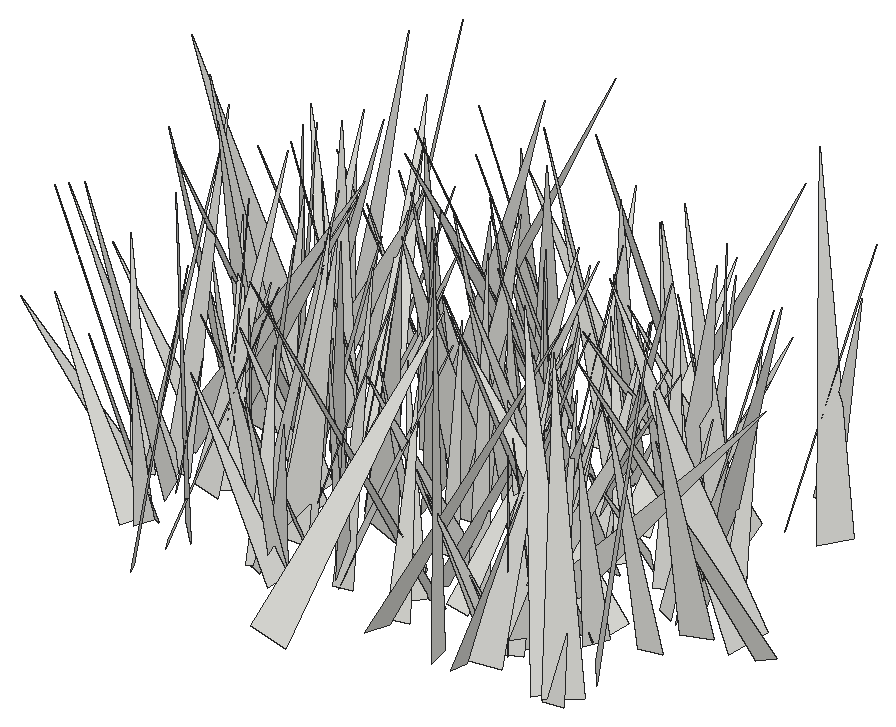
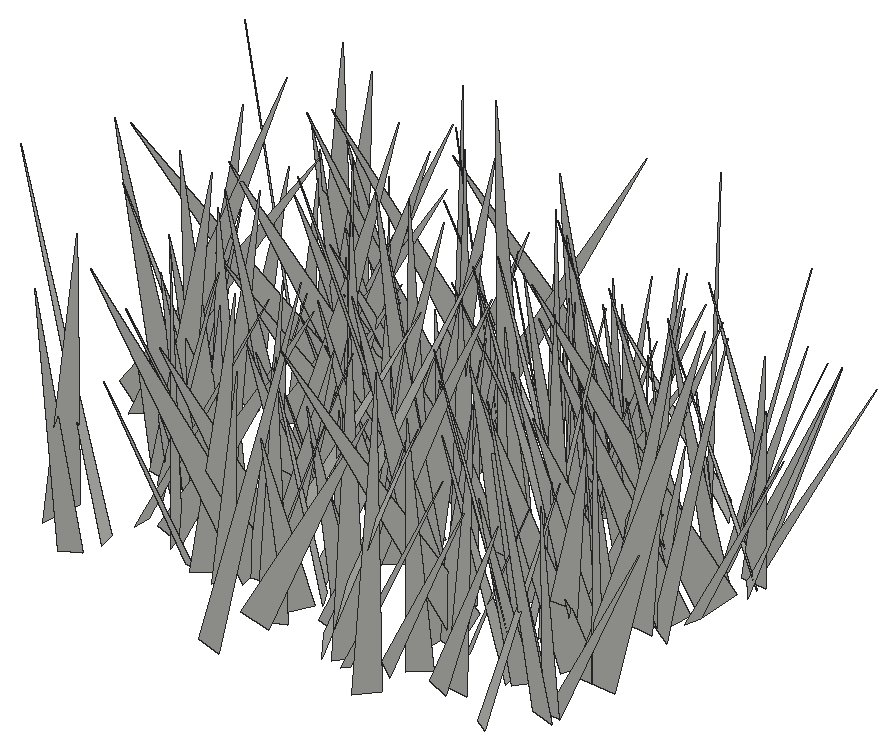
# SketchUp Ruby script. Lengths in inches.
U = 1.inch
M = Sketchup.active_model
def pt(a) = Geom::Point3d.new(a.map { |v| v * U })
def face(e, loops, mat)
  f = e.add_face(loops[0].map { |a| pt(a) })
  loops[1..].each { |l| e.add_face(l.map { |a| pt(a) }).erase! }
  f.material = f.back_material = mat if mat
  f
end
# faces: each face lists its corners as indices into pts; further lists are holes
def faces(e, pts, list, mat = nil) = list.each { |f| face(e, (f[0].is_a?(Array) ? f : [f]).map { |l| l.map { |i| pts[i] } }, mat) }
# xy, xz, yz: faces in a plane at the given z, y or x. An outline is a flat list of corners, or four numbers for a rectangle; further outlines are holes
def ring(l) = l.size == 4 ? [[l[0], l[1]], [l[2], l[1]], [l[2], l[3]], [l[0], l[3]]] : l.each_slice(2).to_a
def flat(e, list, mat, &to3) = list.each { |f| face(e, (f[0].is_a?(Array) ? f : [f]).map { |l| ring(l).map { |u, v| to3.(u, v) } }, mat) }
def xy(e, z, list, mat = nil) = flat(e, list, mat) { |x, y| [x, y, z] }
def xz(e, y, list, mat = nil) = flat(e, list, mat) { |x, z| [x, y, z] }
def yz(e, x, list, mat = nil) = flat(e, list, mat) { |y, z| [x, y, z] }
def lines(e, pts, list) = list.each { |a, b| e.add_line(pt(pts[a]), pt(pts[b])) }
# prism: a flat outline (further loops are holes) pulled along v
def prism(e, loops, v, mat = nil)
  f = face(e, loops, mat); d = Geom::Vector3d.new(v.map { |x| x * U })
  f.pushpull(f.normal.samedirection?(d) ? d.length : -d.length)
end
def box(e, o, s, mat = nil) = prism(e, [[o, [o[0] + s[0], o[1], o[2]], [o[0] + s[0], o[1] + s[1], o[2]], [o[0], o[1] + s[1], o[2]]]], [0, 0, s[2]], mat)
def at(x, y, z, deg = 0) = Geom::Transformation.translation(pt([x, y, z])) * Geom::Transformation.rotation(ORIGIN, Z_AXIS, deg.degrees)
def axes(o, x, y, z) = Geom::Transformation.new([*x, 0, *y, 0, *z, 0, *pt(o).to_a, 1])
def part(name) = M.definitions.add(name)
# library, detail: a bought-in or finely detailed component or shape, given as its bounding box
def library(name, o, s) = part(name).tap { |d| box(d.entities, o, s) }
def detail(e, o, s) = box(e.add_group.entities, o, s)
def put(e, d, t, mat = nil) = e.add_instance(d, t).tap { |i| i.material = mat if mat }
def group(e, t, mat = nil) = e.add_group.tap { |g| g.transformation = t; g.material = mat if mat }.entities
root = M.entities
c1 = part("fur_instance\#9")
p = [[0.8125,0,1.79],[0.67,-0.02,1.48],[0,-0.11,0],[0,0.11,0]]
faces(c1.entities,p,[[0,1,2,3]])
put(root,c1,axes([76.67,339.64,-27.1],[-0.73588,7.38124,0.25307],[6.98236,0.77818,-2.39362],[2.40696,-0.00075,7.02103]))
put(root,c1,axes([69.36,340.53,-27.1],[4.53649,3.63122,1.57008],[3.09166,-4.74451,2.04009],[-2.46831,0.73111,5.44092]))
put(root,c1,axes([74.26,343.21,-27.1],[-4.45422,0.97791,0.2811],[1.01486,4.3608,0.91044],[0.07343,-0.95002,4.4685]))
put(root,c1,axes([73.88,343.84,-27.1],[-3.9744,-0.24759,1.6573],[0.13335,4.20562,0.94807],[1.67038,-0.92483,3.8676]))
put(root,c1,axes([67.49,343.58,-27.1],[2.92591,-1.89098,1.19539],[-1.88086,-3.14489,-0.37117],[-1.21125,0.31559,3.46396]))
put(root,c1,axes([73.47,344.22,-27.1],[0.57309,-4.07864,0.58369],[-4.03575,-0.43699,0.90892],[0.82985,0.69149,4.01716]))
put(root,c1,axes([67.57,344.0625,-27.1],[-2.05359,-3.75931,0.63579],[-3.81243,2.01617,-0.39286],[-0.04503,0.74602,4.26559]))
put(root,c1,axes([88.39,342.84,-27.1],[-4.52139,5.22079,2.42729],[5.56937,4.74843,0.161],[1.45961,-1.94607,6.90462]))
put(root,c1,axes([67.04,343.47,-27.1],[-3.88022,2.75048,0.41463],[2.75578,3.70465,1.21426],[-0.37781,-1.22622,4.59857]))
put(root,c1,axes([69.24,344.07,-27.1],[-4.9247,-5.05159,2.9073],[-5.39927,5.38751,0.21521],[2.19519,1.91829,7.05159]))
put(root,c1,axes([80.1,345.62,-27.1],[-3.80092,-6.72254,0.0507],[-6.48684,3.65215,-2.05545],[-1.76524,1.05421,7.4441]))
put(root,c1,axes([82.68,342.42,-27.1],[-7.45834,-2.27512,2.73301],[-2.96816,7.48025,-1.87304],[1.95846,2.67246,7.56933]))
put(root,c1,axes([84.33,344.62,-27.1],[-3.42009,-2.62307,1.97794],[-2.56254,3.91671,0.76324],[2.05575,0.51835,4.24205]))
put(root,c1,axes([87.82,342.95,-27.1],[-6.04844,4.67756,1.28768],[4.75602,6.12308,0.0974],[0.95811,-0.86582,7.6455]))
put(root,c1,axes([75.96,345.09,-27.1],[3.91592,-0.46866,0.80636],[-0.26131,-3.89224,-0.99321],[-0.89531,-0.91384,3.81675]))
put(root,c1,axes([84.44,343.05,-27.1],[-2.07384,5.25709,1.74566],[5.26815,2.4479,-1.11335],[1.712,-1.16445,5.54061]))
put(root,c1,axes([88.37,342.28,-27.1],[1.19098,5.93826,0.851],[5.76454,-1.37303,1.51343],[-1.66049,-0.50738,5.86438]))
put(root,c1,axes([82.39,345.78,-27.1],[-3.37943,-0.96857,0.84627],[-0.6019,3.29348,1.36586],[1.13667,-1.13567,3.23931]))
put(root,c1,axes([73,343.66,-27.1],[-1.62337,4.08317,1.17277],[4.21606,1.70273,-0.09236],[0.52201,-1.05424,4.39307]))
put(root,c1,axes([82.14,345.75,-27.1],[0.37183,-3.94608,0.38846],[-3.8933,-0.43727,-0.71534],[-0.75144,0.31297,3.89847]))
put(root,c1,axes([65.42,346.04,-27.1],[-4.70731,-0.314,0.0439],[-0.28456,4.4722,1.47573],[0.13983,-1.46975,4.48103]))
put(root,c1,axes([79.5,342.71,-27.1],[7.73901,0.54751,0.09462],[0.50511,-7.48314,1.98706],[-0.23147,1.9758,7.49957]))
put(root,c1,axes([83.77,342.3125,-27.1],[6.82922,2.21825,1.16198],[1.82522,-6.72015,2.10172],[-1.71447,1.68168,6.86597]))
put(root,c1,axes([79.75,343.66,-27.1],[-0.43977,4.5707,0.64422],[4.59918,0.3789,0.45132],[-0.39225,-0.6818,4.56957]))
put(root,c1,axes([69.25,342.79,-27.1],[4.51704,3.2359,0.24642],[3.07452,-4.40221,1.45028],[-1.0388,1.04161,5.3639]))
put(root,c1,axes([66.73,346.16,-27.1],[-6.28754,-2.52373,1.27093],[-2.51372,6.41179,0.29625],[1.29062,0.19325,6.76865]))
put(root,c1,axes([75.96,344.84,-27.1],[4.98455,3.49636,0.32674],[3.50629,-4.92427,-0.79656],[0.19289,-0.83908,6.03621]))
put(root,c1,axes([88.13,345.15,-27.1],[5.88152,4.86813,2.28116],[5.13014,-6.09312,-0.22398],[-1.60749,-1.63397,7.63157]))
put(root,c1,axes([71.04,346.38,-27.1],[-4.89796,-0.50596,1.28828],[-0.38248,5.0478,0.52832],[1.33018,-0.4116,4.8956]))
put(root,c1,axes([66.65,346.67,-27.1],[3.46775,1.51161,0.84573],[1.722,-3.21287,-1.3182],[-0.18693,-1.55498,3.54578]))
put(root,c1,axes([72.72,346.24,-27.1],[2.84119,-6.18581,2.36185],[-6.62137,-2.65127,1.02137],[0.00779,2.57322,6.73004]))
put(root,c1,axes([75.22,345.87,-27.1],[1.82668,3.73793,1.95155],[3.99067,-2.21946,0.51574],[-1.36206,-1.48974,4.1283]))
put(root,c1,axes([84.125,346.46,-27.1],[-3.08736,-2.6391,1.38175],[-2.74426,3.29386,0.15946],[1.15895,0.7691,4.05847]))
put(root,c1,axes([72.91,343.4375,-27.1],[4.10406,6.33899,0.98584],[6.11766,-4.2195,1.66374],[-1.93105,0.10466,7.36601]))
put(root,c1,axes([73.32,346.04,-27.1],[-3.16767,-3.69393,0.44061],[-3.42422,2.66901,-2.24153],[-1.45395,1.76199,4.31912]))
put(root,c1,axes([86.07,347.09,-27.1],[-4.08084,-6.31933,0.93728],[-6.28934,3.77891,-1.90517],[-1.12095,1.80323,7.27719]))
put(root,c1,axes([78.36,346.8,-27.1],[-4.55771,-1.35516,1.4154],[-1.26006,4.77117,0.51063],[1.50069,-0.10962,4.72742]))
put(root,c1,axes([79.8125,348.23,-27.1],[1.26749,-5.25605,0.55346],[-5.00773,-1.37633,-1.60227],[-1.68968,0.13629,5.16385]))
put(root,c1,axes([84.64,344.8125,-27.1],[4.97283,-0.90694,1.68915],[-1.45035,-4.85051,1.66547],[-1.25389,2.01364,4.77261]))
put(root,c1,axes([86.66,347,-27.1],[3.6689,-2.8215,1.45683],[-2.81207,-3.92099,-0.512],[-1.47496,0.45716,4.59995]))
put(root,c1,axes([78.65,344.84,-27.1],[5.2038,5.70361,2.35891],[5.67233,-5.63566,1.11317],[-2.43315,-0.93989,7.64013]))
put(root,c1,axes([82.17,348.57,-27.1],[1.01842,-6.5564,0.3467],[-5.92672,-0.76709,2.90332],[2.82498,0.75429,5.9661]))
put(root,c1,axes([74.91,348.68,-27.1],[-0.13317,-8.12567,1.45261],[-7.87911,0.55826,2.40046],[2.46092,1.34765,7.76415]))
put(root,c1,axes([76.51,344.35,-27.1],[1.43264,6.02249,0.66756],[5.77311,-1.565,1.72927],[-1.84042,-0.22107,5.94411]))
put(root,c1,axes([79.24,345.34,-27.1],[-4.35702,1.54483,0.37411],[1.45493,4.3157,-0.87633],[0.64002,0.7059,4.53896]))
put(root,c1,axes([84.7,344.26,-27.1],[-5.37291,2.30629,0.61766],[1.96946,5.14098,-2.06404],[1.34972,1.6793,5.47055]))
put(root,c1,axes([65.08,346.9,-27.1],[-4.61833,-3.74237,0.73758],[-3.79853,4.40694,-1.4242],[-0.34716,1.56584,5.77113]))
put(root,c1,axes([84.61,346.72,-27.1],[2.40837,2.51325,1.53163],[2.71206,-2.66382,0.10655],[-1.14326,-1.0248,3.47927]))
put(root,c1,axes([72.71,346.01,-27.1],[-0.45657,6.34549,1.8425],[6.59681,0.54314,-0.23589],[0.37708,-1.81886,6.35752]))
put(root,c1,axes([66.14,347.15,-27.1],[-6.00367,-1.40851,0.07652],[-1.40991,5.98159,-0.51624],[-0.04369,0.52005,6.14503]))
put(root,c1,axes([71.98,348.5,-27.1],[-4.35378,0.44066,1.23045],[0.84047,4.2213,1.46212],[1.0009,-1.62788,4.12453]))
put(root,c1,axes([69.75,347.32,-27.1],[3.22406,2.21993,1.84513],[2.48282,-3.54361,-0.0749],[-1.47248,-1.11442,3.91371]))
put(root,c1,axes([88.67,347.77,-27.1],[-0.10037,-5.00985,1.67679],[-5.24561,-0.10471,-0.62683],[-0.62754,1.67652,4.9715]))
put(root,c1,axes([86.66,347.95,-27.1],[-6.39943,2.86094,0.01202],[2.71801,6.07041,2.2137],[-0.89308,-2.0256,6.65111]))
put(root,c1,axes([83.79,345.47,-27.1],[5.89458,-2.32049,1.52507],[-2.76984,-5.16651,2.8446],[-0.1962,3.22166,5.6603]))
put(root,c1,axes([65.08,346.52,-27.1],[-0.91318,4.58049,0.90258],[4.61205,0.74242,0.89849],[-0.72428,-1.04754,4.5834]))
put(root,c1,axes([80.95,345.74,-27.1],[-0.63847,4.33122,0.11328],[4.14955,0.64421,-1.24344],[1.2464,0.07394,4.19773]))
put(root,c1,axes([83.72,346.46,-27.1],[6.0984,-4.54505,0.22334],[-3.82324,-4.91501,4.37303],[2.46783,3.61705,6.22291]))
put(root,c1,axes([82.7,348.18,-27.1],[-2.40754,3.72637,1.88833],[4.14407,2.40561,0.53634],[0.52762,-1.89079,4.40391]))
put(root,c1,axes([79.36,346.64,-27.1],[5.44463,0.12063,0.24069],[0.04962,-5.23956,1.50366],[-0.26462,1.49964,5.23426]))
put(root,c1,axes([89.36,349.72,-27.1],[1.80262,-6.00522,1.15434],[-6.08405,-1.88243,-0.2921],[-0.61598,1.01901,6.26312]))
put(root,c1,axes([69.51,347.91,-27.1],[5.12051,1.66894,1.66295],[1.70709,-5.37015,0.13306],[-1.62376,-0.38277,5.38398]))
put(root,c1,axes([83.625,349.86,-27.1],[-0.04463,-6.97717,1.39975],[-6.92736,-0.27772,-1.60522],[-1.62845,1.37265,6.79015]))
put(root,c1,axes([80.7,347.34,-27.1],[1.55743,6.34801,1.89562],[6.44853,-1.89902,1.06134],[-1.51893,-1.55328,6.44953]))
put(root,c1,axes([69.49,348.87,-27.1],[3.75751,0.05108,0.3502],[0.07903,-3.76142,-0.29936],[-0.34497,-0.30538,3.74592]))
put(root,c1,axes([65.375,346.12,-27.1],[4.3588,4.87451,1.02077],[4.50794,-4.43827,1.9448],[-2.11691,0.58556,6.24322]))
put(root,c1,axes([92.48,350.04,-27.1],[-2.35699,-6.63901,0.53799],[-6.01099,1.87426,-3.2057],[-2.86948,1.52709,6.27339]))
put(root,c1,axes([67.8,346.96,-27.1],[1.8777,6.7714,0.98346],[6.8334,-1.90815,0.09124],[-0.35155,-0.923,7.02632]))
put(root,c1,axes([84.88,349.71,-27.1],[-2.69174,-3.80387,0.07847],[-3.66679,2.56798,-1.29661],[-1.01502,0.8106,4.47591]))
put(root,c1,axes([73.19,347.76,-27.1],[3.15484,4.86518,0.39731],[4.85003,-3.07066,-0.91053],[0.55227,-0.82578,5.72659]))
put(root,c1,axes([71.21,349.74,-27.1],[5.75664,2.23558,0.62086],[2.31995,-5.52205,-1.62697],[0.03364,-1.74108,5.95732]))
put(root,c1,axes([67.2,348.85,-27.1],[-4.37143,-2.8181,2.86453],[-3.24687,4.97094,-0.06453],[2.3675,1.61389,5.20067]))
put(root,c1,axes([83.4,347.96,-27.1],[1.4103,3.34023,0.25009],[3.32818,-1.428,0.30438],[-0.37801,-0.11091,3.61295]))
put(root,c1,axes([70.47,351.62,-27.1],[-2.5118,-6.70095,1.69222],[-6.07027,2.9998,2.86854],[3.30427,0.41708,6.55616]))
put(root,c1,axes([69.82,350.84,-27.1],[0.42063,-4.67833,0.35233],[-4.37367,-0.26302,1.72907],[1.69763,0.48155,4.36738]))
put(root,c1,axes([91.18,350.57,-27.1],[-7.69272,2.37823,1.5322],[2.71051,7.46743,2.01798],[0.8104,-2.40066,7.79498]))
put(root,c1,axes([83.34,351.62,-27.1],[-0.92127,-7.60318,0.93237],[-7.64439,0.85236,-0.60268],[-0.49091,0.99576,7.63504]))
put(root,c1,axes([71.22,349.92,-27.1],[-4.01235,0.08097,0.58825],[0.14386,4.03101,0.42638],[0.5761,-0.44265,3.99045]))
put(root,c1,axes([66.02,347.45,-27.1],[1.84085,7.01016,1.12106],[6.97031,-2.00445,1.08846],[-1.34679,-0.79226,7.16563]))
put(root,c1,axes([78.15,348.76,-27.1],[0.81104,4.54834,1.26147],[4.65262,-0.98593,0.56355],[-0.7949,-1.13006,4.58559]))
put(root,c1,axes([82.19,349.85,-27.1],[3.78368,4.97369,3.03573],[5.56614,-4.15585,-0.12867],[-1.72376,-2.50217,6.24798]))
put(root,c1,axes([68.58,347.65,-27.1],[-4.8792,2.06982,0.10093],[1.96371,4.70056,-1.46614],[0.66196,1.31208,5.09325]))
put(root,c1,axes([73.58,350,-27.1],[4.19942,-1.36084,1.21546],[-1.38514,-4.36301,-0.09922],[-1.1877,0.2767,4.41329]))
put(root,c1,axes([65.04,350.28,-27.1],[-4.32306,0.06447,0.02072],[0.06687,4.27292,0.65655],[0.01068,-0.65679,4.2734]))
put(root,c1,axes([74.94,351.86,-27.1],[7.73874,0.04549,1.82687],[0.5794,-7.60007,-2.26513],[-1.73315,-2.33761,7.39995]))
put(root,c1,axes([82.67,347.84,-27.1],[5.53562,0.75174,0.06867],[0.66774,-5.11345,2.14935],[-0.35205,2.12143,5.1564]))
put(root,c1,axes([75.98,353.14,-27.1],[6.63906,-4.24471,1.17982],[-3.75911,-6.57064,-2.48644],[-2.29753,-1.51516,7.47745]))
put(root,c1,axes([65.96,350.52,-27.1],[1.53162,3.70831,1.75315],[4.01532,-0.97314,-1.44953],[0.83802,-2.1148,3.74116]))
put(root,c1,axes([67.28,349.63,-27.1],[0.68239,3.8164,1.4602],[3.78451,-1.14857,1.23331],[-1.54098,-1.13076,3.67553]))
put(root,c1,axes([64.98,348.79,-27.1],[6.90826,-2.9112,0.5406],[-2.88435,-6.30625,2.89882],[0.66922,2.87186,6.91346]))
put(root,c1,axes([82.61,348.68,-27.1],[-6.55431,0.09701,1.7896],[-0.34688,6.588,-1.62754],[1.75834,1.66126,6.34976]))
put(root,c1,axes([88,352.11,-27.1],[-4.12038,-2.11418,1.50488],[-1.47976,4.23386,1.89649],[2.13184,-1.14743,4.225]))
put(root,c1,axes([71.97,349.47,-27.1],[3.98122,4.30027,2.75674],[4.211,-4.74141,1.31475],[-2.89126,-0.98426,5.71085]))
put(root,c1,axes([77.15,351.37,-27.1],[2.1882,-4.93746,0.79161],[-4.93819,-1.99768,1.19031],[0.78701,1.19336,5.26781]))
put(root,c1,axes([80.67,350.02,-27.1],[-3.32037,-5.8988,2.51801],[-6.36421,2.67847,-2.11746],[-0.7956,3.19234,6.42939]))
put(root,c1,axes([66.33,352.02,-27.1],[-0.95753,-7.17721,1.84222],[-7.39469,1.0444,0.22542],[0.47406,1.79439,7.23729]))
put(root,c1,axes([84.38,353.23,-27.1],[-2.58943,-3.13022,0.07236],[-2.65217,2.2427,2.10831],[1.66419,-1.2964,3.47253]))
put(root,c1,axes([73.65,348.23,-27.1],[5.66789,4.81372,1.80284],[4.22946,-5.89252,2.43659],[-2.92126,0.80836,7.02566]))
put(root,c1,axes([68.09,352.68,-27.1],[-3.16334,-6.14078,0.476],[-6.132,3.08971,-0.89149],[-0.57823,0.82883,6.8499]))
put(root,c1,axes([87.19,351.77,-27.1],[2.31724,-3.70248,0.25487],[-3.62607,-2.19471,1.08527],[0.79054,0.78602,4.23086]))
put(root,c1,axes([65.41,351.78,-27.1],[-3.32824,-5.52708,1.61735],[-5.74671,3.30884,-0.51825],[0.37393,1.65668,6.43096]))
put(root,c1,axes([87.33,350.34,-27.1],[1.79566,3.71313,0.76849],[3.77743,-1.82574,-0.00496],[-0.33004,-0.69403,4.12452]))
put(root,c1,axes([77.35,351.26,-27.1],[5.13352,5.29295,1.04527],[5.31008,-4.70157,-2.27141],[0.95446,-2.31104,7.01492]))
put(root,c1,axes([68.92,352.63,-27.1],[5.69332,3.04756,1.30745],[3.31373,-5.12843,-2.47574],[0.12746,-2.79687,5.96424]))
put(root,c1,axes([65.43,350.87,-27.1],[6.30652,-2.10429,0.15189],[-2.07978,-6.12031,1.56194],[0.35446,1.52876,6.46224]))
put(root,c1,axes([76.74,352.23,-27.1],[1.64053,-3.56149,0.70323],[-3.59089,-1.47867,0.88831],[0.53314,0.99969,3.81922]))
put(root,c1,axes([66.89,352.72,-27.1],[6.73753,-0.02978,4.19134],[0.53715,-7.86314,-0.91932],[-4.15689,-1.06433,6.67458]))
put(root,c1,axes([78.25,352.61,-27.1],[4.81176,-1.3762,1.70282],[-1.26945,-5.10354,-0.53746],[-1.78382,-0.0803,4.97575]))
put(root,c1,axes([86.23,351.98,-27.1],[-2.39493,4.93051,2.15105],[5.27679,2.61079,-0.10925],[1.04521,-1.88321,5.4803]))
put(root,c1,axes([87.83,350.42,-27.1],[5.27233,3.79468,0.9806],[3.62511,-5.34626,1.19781],[-1.48988,0.42019,6.38454]))
put(root,c1,axes([75.34,353.4,-27.1],[0.9927,-7.18833,2.00129],[-7.23058,-0.4281,2.04891],[1.84279,2.19257,6.96128]))
put(root,c1,axes([76.23,351.89,-27.1],[4.34648,-1.55951,0.20323],[-1.53377,-4.07129,1.56122],[0.34774,1.53551,4.34586]))
put(root,c1,axes([84.6,354.58,-27.1],[0.33482,-6.22736,0.74708],[-6.26175,-0.28913,0.39628],[0.3585,0.76592,6.22375]))
put(root,c1,axes([81.875,353.31,-27.1],[6.64605,0.23955,0.93352],[0.28653,-6.70181,-0.32012],[-0.92019,-0.35664,6.64266]))
put(root,c1,axes([72.625,354.61,-27.1],[0.91835,-4.65892,0.5996],[-4.68613,-0.86646,0.44487],[0.32448,0.67241,4.72768]))
put(root,c1,axes([69.25,354.91,-27.1],[-4.71687,-4.84842,1.35584],[-4.8132,4.8877,0.73342],[1.47602,0.44449,6.72444]))
put(root,c1,axes([86.52,354.12,-27.1],[7.28234,-1.08518,0.65082],[-1.04869,-7.30325,-0.44316],[-0.70811,-0.34428,7.3494]))
put(root,c1,axes([82.45,351.84,-27.1],[-3.28423,2.60896,0.74342],[2.31234,3.30268,-1.37511],[1.4186,0.65664,3.96257]))
put(root,c1,axes([83.69,352.53,-27.1],[-4.1604,2.35856,0.20079],[2.33408,4.15517,-0.44576],[0.39395,0.28953,4.76162]))
put(root,c1,axes([85.84,353.4,-27.1],[-2.17723,3.86998,1.04919],[4.00343,2.16477,0.32287],[0.22393,-1.07466,4.42864]))
put(root,c1,axes([68.23,354.43,-27.1],[-4.38219,4.14776,3.28171],[4.71988,4.98997,-0.0042],[2.38668,-2.25242,6.03386]))
put(root,c1,axes([82.37,352.34,-27.1],[-4.0426,1.99311,1.15136],[1.52694,4.06338,-1.67276],[1.72237,1.07573,4.18533]))
put(root,c1,axes([81.2,352.27,-27.1],[1.74005,3.73475,0.21366],[3.48509,-1.70407,1.40429],[-1.35946,0.41179,3.87351]))
put(root,c1,axes([68.85,350.8125,-27.1],[-5.84983,3.65343,0.11485],[3.32744,5.4123,-2.68634],[1.51292,2.22277,6.35229]))
put(root,c1,axes([84.25,355.37,-27.1],[4.71855,-5.46855,1.25045],[-5.59838,-4.69426,0.59612],[-0.35606,1.33873,7.19821]))
put(root,c1,axes([70,354.49,-27.1],[4.56637,-2.19972,0.30987],[-2.21681,-4.46657,0.96025],[0.14341,0.99877,4.97679]))
put(root,c1,axes([65.95,353.96,-27.1],[0.08928,4.21713,1.27448],[4.4055,-0.088,-0.01741],[-0.00879,-1.27457,4.21804]))
put(root,c1,axes([76.69,353.93,-27.1],[-0.20342,5.45726,1.92359],[5.57072,0.70526,-1.41173],[1.56492,-1.80117,5.27542]))
put(root,c1,axes([87.33,354.2,-27.1],[-0.80473,7.1427,2.6366],[7.51279,0.31449,1.44102],[-1.23607,-2.73867,7.04196]))
put(root,c1,axes([66.2,354.45,-27.1],[3.99026,4.07334,2.14881],[4.32029,-4.29562,0.12027],[-1.59518,-1.44473,5.70086]))
put(root,c1,axes([64.88,356.44,-27.1],[1.74253,-7.39949,2.19817],[-7.33714,-2.28781,-1.88496],[-2.39807,1.62304,7.36449]))
put(root,c1,axes([79.17,353.76,-27.1],[-0.87591,3.86506,0.33078],[3.84564,0.82067,0.59405],[-0.50909,-0.4507,3.91829]))
put(root,c1,axes([68.9,354.08,-27.1],[-3.88558,0.60859,0.85055],[0.43871,3.91906,-0.80001],[0.9494,0.67978,3.85072]))
put(root,c1,axes([78.1,356.59,-27.1],[-5.60021,-5.8066,0.30959],[-5.79691,5.54128,-0.92996],[-0.45638,0.8674,8.01337]))
put(root,c1,axes([86.94,355.16,-27.1],[-4.01127,-3.66818,1.32519],[-3.89401,3.87381,-1.06408],[0.2199,1.68524,5.33044]))
put(root,c1,axes([81.21,354.58,-27.1],[-6.43148,-3.95381,0.27263],[-3.76371,5.93049,-2.78112],[-1.24153,2.50351,7.01869]))
put(root,c1,axes([84.63,357.43,-27.1],[0.43766,-5.35462,0.13989],[-4.92597,-0.45748,-2.09965],[-2.10387,-0.04276,4.94519]))
put(root,c1,axes([88.47,353.1,-27.1],[-4.48023,1.71415,0.10108],[1.53614,4.12726,-1.90446],[0.76734,1.74596,4.4027]))
put(root,c1,axes([83.72,354.86,-27.1],[2.80072,3.68056,0.20092],[3.50306,-2.57922,-1.58339],[1.14693,-1.10998,4.34551]))
put(root,c1,axes([66.41,354.64,-27.1],[6.19902,-0.22924,1.58295],[-0.50577,-6.29178,1.06951],[-1.51739,1.16065,6.11037]))
put(root,c1,axes([66.17,355.82,-27.1],[4.35594,-4.3452,0.48537],[-4.22774,-4.01128,2.03138],[1.11472,1.7662,5.80763]))
put(root,c1,axes([71.08,353.2,-27.1],[-3.48559,6.14429,0.41822],[6.11379,3.5101,-0.61419],[0.74073,-0.05879,7.03735]))
put(root,c1,axes([71.57,357.37,-27.1],[-1.87294,-5.65903,1.00828],[-5.62978,2.02003,0.87988],[1.16052,0.66634,5.89562]))
put(root,c1,axes([65.23,355.83,-27.1],[-4.85936,-1.80324,2.4582],[-1.94231,5.39639,0.11902],[2.34986,0.73149,5.18178]))
put(root,c1,axes([76.25,356.07,-27.1],[-3.7574,-4.18768,1.74578],[-4.4509,3.84178,-0.36412],[0.87968,1.55129,5.61445]))
put(root,c1,axes([86.07,357.34,-27.1],[-5.4104,-1.19331,0.05848],[-1.15989,5.3113,1.06983],[0.28647,-1.03242,5.43616]))
put(root,c1,axes([85.44,354.87,-27.1],[5.18015,0.30458,2.40247],[-0.20645,-5.59667,1.15468],[-2.41288,1.13276,5.059]))
put(root,c1,axes([67.82,354.98,-27.1],[-2.82943,5.24506,0.49337],[5.22615,2.72388,1.01368],[-0.66438,-0.91081,5.87271]))
put(root,c1,axes([79.9,358.06,-27.1],[-1.23587,-5.65616,0.92472],[-5.5483,1.41785,1.25724],[1.43652,0.61007,5.65145]))
put(root,c1,axes([75.2,359.29,-27.1],[-0.88458,-7.33954,0.10795],[-7.20369,0.84713,-1.43254],[-1.40973,0.27658,7.25253]))
put(root,c1,axes([67.17,357.29,-27.1],[1.41484,-4.55258,1.06253],[-4.54528,-1.07998,1.42506],[1.09333,1.40157,4.54939]))
put(root,c1,axes([77.49,355.35,-27.1],[3.33394,1.47543,1.26624],[0.9738,-3.44268,1.44745],[-1.68284,0.93087,3.34618]))
put(root,c1,axes([79.76,357.08,-27.1],[0.51311,-4.91857,2.52241],[-5.22585,-1.25725,-1.38854],[-1.80151,2.24614,4.74633]))
put(root,c1,axes([82.46,354.58,-27.1],[-2.9389,4.8588,0.20427],[4.55933,2.83593,-1.85926],[1.6918,0.79774,5.36547]))
put(root,c1,axes([84.16,357.66,-27.1],[5.47086,1.91538,2.35531],[2.21322,-5.83902,-0.39241],[-2.07794,-1.17628,5.78316]))
put(root,c1,axes([69.95,357.86,-27.1],[-3.92921,-1.09616,0.24918],[-1.11465,3.91653,-0.34741],[0.14562,0.40197,4.06442]))
put(root,c1,axes([76.04,357.54,-27.1],[2.99214,-2.75371,1.44433],[-3.06357,-2.95389,0.71483],[-0.53251,1.52102,4.0031]))
put(root,c1,axes([71.57,357.03,-27.1],[7.18053,-1.42617,1.70446],[-1.71997,-7.21687,1.20732],[-1.40743,1.54336,7.22055]))
put(root,c1,axes([76.97,357.64,-27.1],[4.26525,2.34746,1.0733],[2.44325,-4.34035,-0.2164],[-0.83252,-0.71113,4.86375]))
put(root,c1,axes([67.61,358.04,-27.1],[4.85217,1.44436,0.49792],[1.4914,-4.83766,-0.50049],[-0.33141,-0.62336,5.03778]))
put(root,c1,axes([81.73,358.79,-27.1],[3.82096,-4.05561,2.24215],[-4.19487,-4.26194,-0.56033],[-1.96935,1.20949,5.5438]))
put(root,c1,axes([80.11,357.05,-27.1],[-6.83624,-2.0461,0.45627],[-2.08301,6.45462,-2.26447],[-0.23611,2.29788,6.76704]))
put(root,c1,axes([67.02,358.08,-27.1],[2.18192,-3.03993,1.35648],[-3.32882,-1.9865,0.90262],[0.01238,1.6293,3.63142]))
put(root,c1,axes([86.24,359.27,-27.1],[7.20484,3.15988,1.15153],[3.35999,-6.88107,-2.14053],[-0.14588,-2.42624,7.57051]))
put(root,c1,axes([70.7,359.72,-27.1],[2.83156,-3.99697,0.33188],[-4.00855,-2.80696,0.39506],[0.13188,0.49882,4.88236]))
put(root,c1,axes([64.76,358.9,-27.1],[-2.53868,-3.44184,0.53172],[-3.38696,2.28677,-1.36858],[-0.81085,1.22404,4.05193]))
put(root,c1,axes([67.97,357.14,-27.1],[5.71474,5.0925,1.62445],[5.00095,-5.93344,1.00766],[-1.88756,-0.30227,7.58791]))
put(root,c1,axes([74.44,359.84,-27.1],[-1.9055,-4.08481,0.78377],[-4.15591,1.83492,-0.5407],[-0.16841,0.93717,4.47485]))
put(root,c1,axes([68.62,360.08,-27.1],[-1.39495,-5.41554,1.57218],[-5.52882,1.63221,0.71678],[1.10996,1.3242,5.54619]))
put(root,c1,axes([64.71,359.28,-27.1],[-0.60793,-4.00143,1.69165],[-4.28266,0.83877,0.44495],[0.72934,1.58988,4.02282]))
put(root,c1,axes([73.39,360.67,-27.1],[5.78336,-2.78291,1.02515],[-2.6557,-5.85961,-0.92463],[-1.32013,-0.40388,6.35113]))
put(root,c1,axes([82.56,358.8125,-27.1],[2.24479,3.42751,0.35228],[3.3467,-2.06895,-1.19586],[0.81948,-0.93948,3.91878]))
put(root,c1,axes([80.94,358.78,-27.1],[-4.87312,1.26006,1.29377],[1.19613,5.04128,-0.40455],[1.35309,0.08157,5.01711]))
put(root,c1,axes([71.18,356.15,-27.1],[7.74445,1.42991,0.81828],[1.0012,-7.20795,3.11989],[-1.30836,2.94814,7.231]))
put(root,c1,axes([73.08,361.22,-27.1],[-3.99864,-1.03805,0.42764],[-0.78188,3.71014,1.695],[0.80565,-1.55139,3.76744]))
put(root,c1,axes([80.3,357.61,-27.1],[7.35163,-0.33714,0.71191],[-0.54127,-7.01692,2.26646],[-0.57229,2.30568,7.00167]))
put(root,c1,axes([66.24,361.56,-27.1],[-3.01664,-4.03882,0.35129],[-3.9528,3.02747,0.86334],[0.90049,-0.2406,4.96657]))
put(root,c1,axes([77.39,360.28,-27.1],[1.77747,-4.94769,1.74658],[-5.22789,-1.82695,0.145],[-0.44649,1.69476,5.25529]))
put(root,c1,axes([71.75,360.46,-27.1],[-2.18116,-3.44946,0.52539],[-3.41914,1.9894,-1.13316],[-0.6959,1.0372,3.92074]))
put(root,c1,axes([64.84,359.64,-27.1],[2.76981,6.05425,2.08045],[6.39697,-2.70498,-0.64491],[-0.24704,-2.16406,6.62646]))
put(root,c1,axes([69.35,360.32,-27.1],[-0.15517,3.72025,1.9318],[3.94772,-0.52047,1.31942],[-1.40985,-1.86683,3.48188]))
put(root,c1,axes([78.01,360.59,-27.1],[-2.55985,4.83206,1.74885],[4.89019,1.69025,2.4878],[-1.579,-2.59892,4.86955]))
put(root,c1,axes([88.86,358.74,-27.1],[-7.32985,2.37013,1.25415],[2.21242,7.40801,-1.06942],[1.51512,0.64882,7.62892]))
put(root,c1,axes([86.77,360.79,-27.1],[0.64184,-5.02818,1.67754],[-5.1921,-0.25617,1.21871],[1.0672,1.77778,4.9203]))
put(root,c1,axes([71.19,362.3125,-27.1],[5.82388,-2.11588,0.96568],[-1.89422,-5.82584,-1.34106],[-1.34958,-0.95373,6.04946]))
put(root,c1,axes([77.24,358.81,-27.1],[-3.56448,3.67904,0.44666],[3.56023,3.5714,-1.00507],[1.02934,0.38746,5.02301]))
put(root,c1,axes([74.77,360.51,-27.1],[-5.23852,-3.39609,0.6769],[-3.443,4.97658,-1.67721],[-0.37061,1.77027,6.01352]))
put(root,c1,axes([78.14,363.21,-27.1],[-2.86218,-6.85746,0.77217],[-6.83354,2.93291,0.71683],[0.96112,0.43167,7.39614]))
